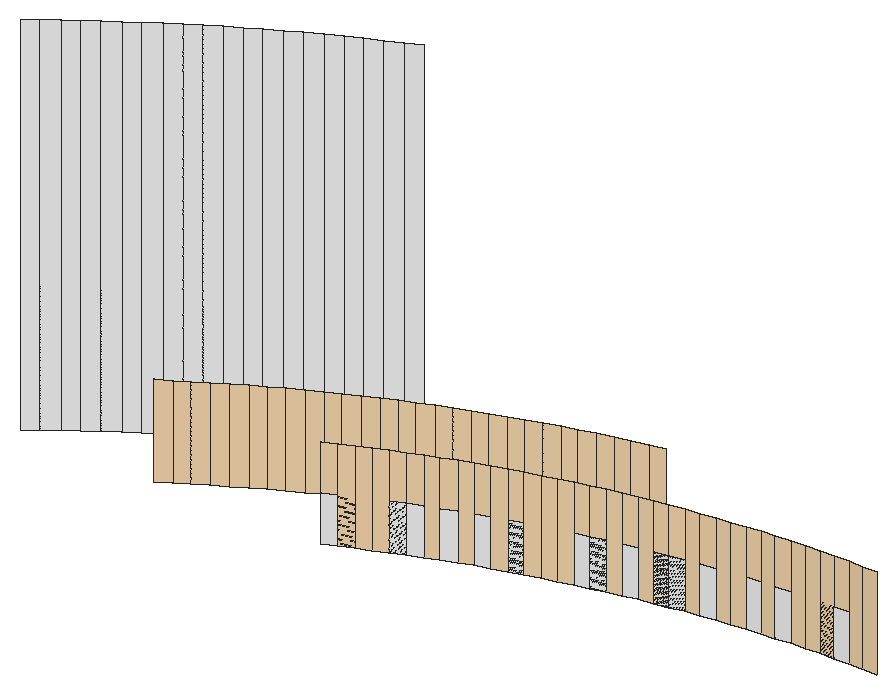
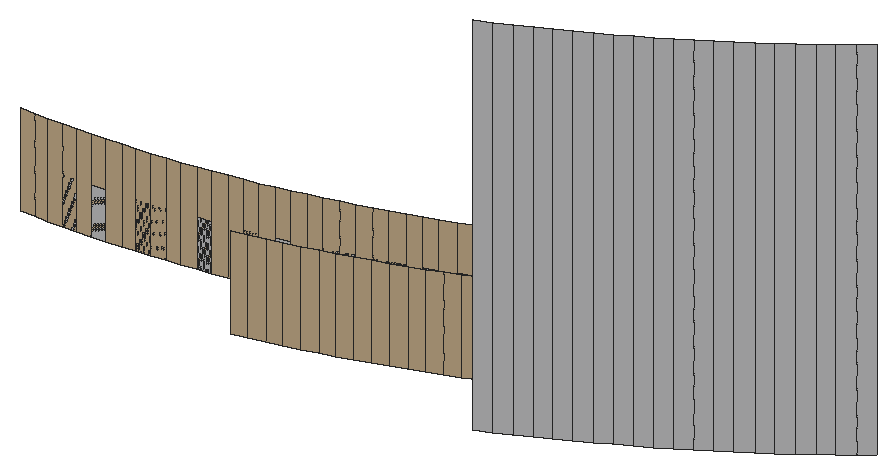
# SketchUp Ruby script. Lengths in inches.
U = 1.inch
M = Sketchup.active_model
def pt(a) = Geom::Point3d.new(a.map { |v| v * U })
def face(e, loops, mat)
  f = e.add_face(loops[0].map { |a| pt(a) })
  loops[1..].each { |l| e.add_face(l.map { |a| pt(a) }).erase! }
  f.material = f.back_material = mat if mat
  f
end
# faces: each face lists its corners as indices into pts; further lists are holes
def faces(e, pts, list, mat = nil) = list.each { |f| face(e, (f[0].is_a?(Array) ? f : [f]).map { |l| l.map { |i| pts[i] } }, mat) }
# xy, xz, yz: faces in a plane at the given z, y or x. An outline is a flat list of corners, or four numbers for a rectangle; further outlines are holes
def ring(l) = l.size == 4 ? [[l[0], l[1]], [l[2], l[1]], [l[2], l[3]], [l[0], l[3]]] : l.each_slice(2).to_a
def flat(e, list, mat, &to3) = list.each { |f| face(e, (f[0].is_a?(Array) ? f : [f]).map { |l| ring(l).map { |u, v| to3.(u, v) } }, mat) }
def xy(e, z, list, mat = nil) = flat(e, list, mat) { |x, y| [x, y, z] }
def xz(e, y, list, mat = nil) = flat(e, list, mat) { |x, z| [x, y, z] }
def yz(e, x, list, mat = nil) = flat(e, list, mat) { |y, z| [x, y, z] }
def lines(e, pts, list) = list.each { |a, b| e.add_line(pt(pts[a]), pt(pts[b])) }
# prism: a flat outline (further loops are holes) pulled along v
def prism(e, loops, v, mat = nil)
  f = face(e, loops, mat); d = Geom::Vector3d.new(v.map { |x| x * U })
  f.pushpull(f.normal.samedirection?(d) ? d.length : -d.length)
end
def box(e, o, s, mat = nil) = prism(e, [[o, [o[0] + s[0], o[1], o[2]], [o[0] + s[0], o[1] + s[1], o[2]], [o[0], o[1] + s[1], o[2]]]], [0, 0, s[2]], mat)
def at(x, y, z, deg = 0) = Geom::Transformation.translation(pt([x, y, z])) * Geom::Transformation.rotation(ORIGIN, Z_AXIS, deg.degrees)
def axes(o, x, y, z) = Geom::Transformation.new([*x, 0, *y, 0, *z, 0, *pt(o).to_a, 1])
def part(name) = M.definitions.add(name)
# library, detail: a bought-in or finely detailed component or shape, given as its bounding box
def library(name, o, s) = part(name).tap { |d| box(d.entities, o, s) }
def detail(e, o, s) = box(e.add_group.entities, o, s)
def put(e, d, t, mat = nil) = e.add_instance(d, t).tap { |i| i.material = mat if mat }
def group(e, t, mat = nil) = e.add_group.tap { |g| g.transformation = t; g.material = mat if mat }.entities
root = M.entities
M.materials.add("False Ceiling Light").color = [254, 223, 179]
M.materials.add("[Quartz Light Grey]").color = [251, 251, 252]
xz(root,217.5,[[56.65,115.32,56.82,116.49],[56.82,115.32,57,116.49]],"False Ceiling Light")
xz(root,217.5,[[56.65,115.32,56.82,115.91],[56.82,115.32,57,115.91]],"[Quartz Light Grey]")
p = [[47.25,216.05,115.32],[47.4,216.17,115.32],[47.4,216.17,120],[47.25,216.05,120],[49.1,216.16,115.32],[48.94,216.06,115.32],
  [48.94,216.06,116.49],[49.1,216.16,116.49],[51.03,216.11,115.32],[51.1875,216.18,115.32],[51.1875,216.18,116.49],[51.03,216.11,116.49],
  [51.1875,216.18,115.32],[51.03,216.11,115.32],[51.03,216.11,115.91],[51.1875,216.18,115.91],[47.5625,216.3,115.32],[47.5625,216.3,120],
  [49.26,216.26,115.32],[49.26,216.26,116.49],[51.35,216.26,115.32],[51.35,216.26,116.49],[51.35,216.26,115.32],[51.35,216.26,115.91],
  [47.73,216.42,115.32],[47.73,216.42,120],[49.42,216.36,115.32],[49.42,216.36,116.49],[51.51,216.33,115.32],[51.51,216.33,116.49],
  [51.51,216.33,115.32],[51.51,216.33,115.91],[51.67,216.4,115.32],[51.67,216.4,116.49],[51.67,216.4,115.32],[51.67,216.4,115.91],
  [47.89,216.54,115.32],[47.89,216.54,120],[49.59,216.46,115.32],[49.59,216.46,116.49],[51.83,216.47,115.32],[51.83,216.47,116.49],
  [51.83,216.47,115.32],[51.83,216.47,115.91],[48.05,216.66,115.32],[48.05,216.66,120],[49.75,216.56,115.32],[49.75,216.56,116.49],
  [52,216.54,115.32],[52,216.54,116.49],[52,216.54,115.32],[52,216.54,115.91],[52.16,216.6,115.32],[52.16,216.6,116.49],
  [52.16,216.6,115.32],[52.16,216.6,115.91],[49.91,216.65,115.32],[49.91,216.65,116.49],[52.33,216.67,115.32],[52.33,216.67,116.49],
  [52.33,216.67,115.32],[52.33,216.67,115.91],[48.22,216.77,115.32],[48.22,216.77,120],[50.08,216.74,115.32],[50.08,216.74,116.49],
  [50.25,216.83,115.32],[50.25,216.83,116.49],[52.49,216.73,115.32],[52.49,216.73,116.49],[52.49,216.73,115.32],[52.49,216.73,115.91],
  [52.66,216.78,115.32],[52.66,216.78,116.49],[52.66,216.78,115.32],[52.66,216.78,115.91],[48.39,216.89,115.32],[48.39,216.89,120],
  [50.42,216.92,115.32],[50.42,216.92,116.49],[52.83,216.84,115.32],[52.83,216.84,116.49],[52.83,216.84,115.32],[52.83,216.84,115.91],
  [53,216.89,115.32],[53,216.89,116.49],[53,216.89,115.32],[53,216.89,115.91],[48.56,217,115.32],[48.56,217,120],
  [50.59,217,115.32],[50.59,217,116.49],[53.17,216.94,115.32],[53.17,216.94,116.49],[53.17,216.94,115.32],[53.17,216.94,115.91],
  [53.34,216.99,115.32],[53.34,216.99,116.49],[53.34,216.99,115.32],[53.34,216.99,115.91],[48.73,217.11,115.32],[48.73,217.11,120],
  [50.76,217.09,115.32],[50.76,217.09,116.49],[53.51,217.04,115.32],[53.51,217.04,116.49],[53.51,217.04,115.32],[53.51,217.04,115.91],
  [53.68,217.08,115.32],[53.68,217.08,116.49],[53.68,217.08,115.32],[53.68,217.08,115.91],[48.9,217.22,115.32],[48.9,217.22,120],
  [50.93,217.17,115.32],[50.93,217.17,116.49],[53.85,217.13,115.32],[53.85,217.13,116.49],[53.85,217.13,115.32],[53.85,217.13,115.91],
  [54.02,217.17,115.32],[54.02,217.17,116.49],[54.02,217.17,115.32],[54.02,217.17,115.91],[49.07,217.32,115.32],[49.07,217.32,120],
  [51.1,217.25,115.32],[51.1,217.25,116.49],[51.28,217.32,115.32],[51.28,217.32,116.49],[54.19,217.21,115.32],[54.19,217.21,116.49],
  [54.19,217.21,115.32],[54.19,217.21,115.91],[54.37,217.24,115.32],[54.37,217.24,116.49],[54.37,217.24,115.32],[54.37,217.24,115.91],
  [54.54,217.27,115.32],[54.54,217.27,116.49],[54.54,217.27,115.32],[54.54,217.27,115.91],[49.25,217.42,115.32],[49.25,217.42,120],
  [51.45,217.4,115.32],[51.45,217.4,116.49],[54.71,217.31,115.32],[54.71,217.31,116.49],[54.71,217.31,115.32],[54.71,217.31,115.91],
  [54.89,217.33,115.32],[54.89,217.33,116.49],[54.89,217.33,115.32],[54.89,217.33,115.91],[55.0625,217.36,115.32],[55.0625,217.36,116.49],
  [55.0625,217.36,115.32],[55.0625,217.36,115.91],[49.43,217.52,115.32],[49.43,217.52,120],[51.625,217.47,115.32],[51.625,217.47,116.49],
  [55.24,217.38,115.32],[55.24,217.38,116.49],[55.24,217.38,115.32],[55.24,217.38,115.91],[55.41,217.41,115.32],[55.41,217.41,116.49],
  [55.41,217.41,115.32],[55.41,217.41,115.91],[55.59,217.43,115.32],[55.59,217.43,116.49],[55.59,217.43,115.32],[55.59,217.43,115.91],
  [55.76,217.44,115.32],[55.76,217.44,116.49],[55.76,217.44,115.32],[55.76,217.44,115.91],[55.94,217.46,115.32],[55.94,217.46,116.49],
  [55.94,217.46,115.32],[55.94,217.46,115.91],[49.6,217.62,115.32],[49.6,217.62,120],[51.8,217.54,115.32],[51.8,217.54,116.49],
  [51.98,217.6,115.32],[51.98,217.6,116.49],[56.12,217.47,115.32],[56.12,217.47,116.49],[56.12,217.47,115.32],[56.12,217.47,115.91],
  [56.29,217.48,115.32],[56.29,217.48,116.49],[56.29,217.48,115.32],[56.29,217.48,115.91],[56.47,217.49,115.32],[56.47,217.49,116.49],
  [56.47,217.49,115.32],[56.47,217.49,115.91],[56.65,217.5,115.32],[56.65,217.5,116.49],[56.65,217.5,115.32],[56.65,217.5,115.91],
  [49.78,217.72,115.32],[49.78,217.72,120],[52.16,217.67,115.32],[52.16,217.67,116.49],[49.96,217.8125,115.32],[49.96,217.8125,120],
  [52.34,217.73,115.32],[52.34,217.73,116.49],[52.52,217.79,115.32],[52.52,217.79,116.49],[50.14,217.9,115.32],[50.14,217.9,120],
  [52.7,217.85,115.32],[52.7,217.85,116.49],[52.88,217.9,115.32],[52.88,217.9,116.49],[50.33,217.99,115.32],[50.33,217.99,120],
  [53.0625,217.96,115.32],[53.0625,217.96,116.49],[50.51,218.08,115.32],[50.51,218.08,120],[53.25,218.01,115.32],[53.25,218.01,116.49],
  [53.43,218.05,115.32],[53.43,218.05,116.49],[50.7,218.16,115.32],[50.7,218.16,120],[53.62,218.1,115.32],[53.62,218.1,116.49],
  [53.8,218.14,115.32],[53.8,218.14,116.49]]
faces(root,p,[[0,1,2,3],[12,13,14,15],[1,16,17,2],[22,12,15,23],[16,24,25,17],[30,22,23,31],[34,30,31,35],[24,36,37,25],
  [42,34,35,43],[36,44,45,37],[50,42,43,51],[54,50,51,55],[60,54,55,61],[44,62,63,45],[70,60,61,71],[74,70,71,75],
  [62,76,77,63],[82,74,75,83],[86,82,83,87],[76,88,89,77],[94,86,87,95],[98,94,95,99],[88,100,101,89],[106,98,99,107],
  [110,106,107,111],[100,112,113,101],[118,110,111,119],[122,118,119,123],[112,124,125,113],[132,122,123,133],[136,132,133,137],[140,136,137,141],
  [124,142,143,125],[148,140,141,149],[152,148,149,153],[156,152,153,157],[142,158,159,143],[164,156,157,165],[168,164,165,169],[172,168,169,173],
  [176,172,173,177],[180,176,177,181],[158,182,183,159],[190,180,181,191],[194,190,191,195],[198,194,195,199],[202,198,199,203],[182,204,205,183],
  [204,208,209,205],[208,214,215,209],[214,220,221,215],[220,224,225,221],[224,230,231,225]],"[Quartz Light Grey]")
faces(root,p,[[4,5,6,7],[8,9,10,11],[18,4,7,19],[9,20,21,10],[26,18,19,27],[20,28,29,21],[28,32,33,29],[38,26,27,39],
  [32,40,41,33],[46,38,39,47],[40,48,49,41],[48,52,53,49],[56,46,47,57],[52,58,59,53],[64,56,57,65],[66,64,65,67],
  [58,68,69,59],[68,72,73,69],[78,66,67,79],[72,80,81,73],[80,84,85,81],[90,78,79,91],[84,92,93,85],[92,96,97,93],
  [102,90,91,103],[96,104,105,97],[104,108,109,105],[114,102,103,115],[108,116,117,109],[116,120,121,117],[126,114,115,127],[128,126,127,129],
  [120,130,131,121],[130,134,135,131],[134,138,139,135],[144,128,129,145],[138,146,147,139],[146,150,151,147],[150,154,155,151],[160,144,145,161],
  [154,162,163,155],[162,166,167,163],[166,170,171,167],[170,174,175,171],[174,178,179,175],[184,160,161,185],[186,184,185,187],[178,188,189,179],
  [188,192,193,189],[192,196,197,193],[196,200,201,197],[206,186,187,207],[210,206,207,211],[212,210,211,213],[216,212,213,217],[218,216,217,219],
  [222,218,219,223],[226,222,223,227],[228,226,227,229],[232,228,229,233],[234,232,233,235]],"False Ceiling Light")
